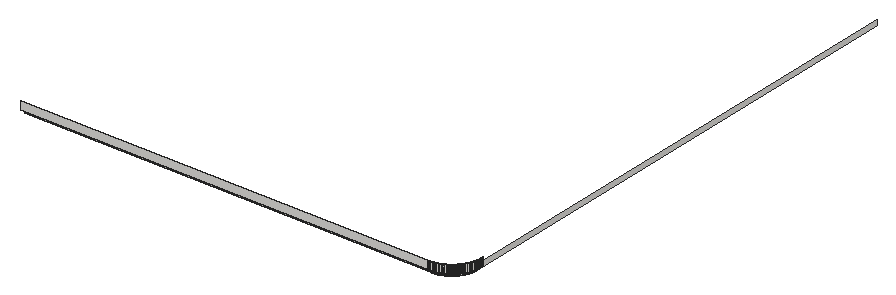
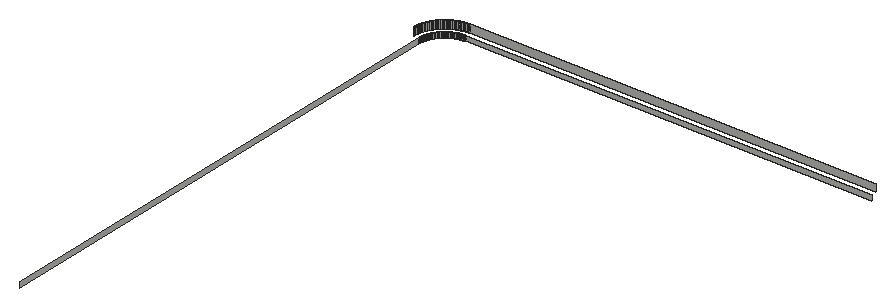
# SketchUp Ruby script. Lengths in inches.
U = 1.inch
M = Sketchup.active_model
def pt(a) = Geom::Point3d.new(a.map { |v| v * U })
def face(e, loops, mat)
  f = e.add_face(loops[0].map { |a| pt(a) })
  loops[1..].each { |l| e.add_face(l.map { |a| pt(a) }).erase! }
  f.material = f.back_material = mat if mat
  f
end
# faces: each face lists its corners as indices into pts; further lists are holes
def faces(e, pts, list, mat = nil) = list.each { |f| face(e, (f[0].is_a?(Array) ? f : [f]).map { |l| l.map { |i| pts[i] } }, mat) }
# xy, xz, yz: faces in a plane at the given z, y or x. An outline is a flat list of corners, or four numbers for a rectangle; further outlines are holes
def ring(l) = l.size == 4 ? [[l[0], l[1]], [l[2], l[1]], [l[2], l[3]], [l[0], l[3]]] : l.each_slice(2).to_a
def flat(e, list, mat, &to3) = list.each { |f| face(e, (f[0].is_a?(Array) ? f : [f]).map { |l| ring(l).map { |u, v| to3.(u, v) } }, mat) }
def xy(e, z, list, mat = nil) = flat(e, list, mat) { |x, y| [x, y, z] }
def xz(e, y, list, mat = nil) = flat(e, list, mat) { |x, z| [x, y, z] }
def yz(e, x, list, mat = nil) = flat(e, list, mat) { |y, z| [x, y, z] }
def lines(e, pts, list) = list.each { |a, b| e.add_line(pt(pts[a]), pt(pts[b])) }
# prism: a flat outline (further loops are holes) pulled along v
def prism(e, loops, v, mat = nil)
  f = face(e, loops, mat); d = Geom::Vector3d.new(v.map { |x| x * U })
  f.pushpull(f.normal.samedirection?(d) ? d.length : -d.length)
end
def box(e, o, s, mat = nil) = prism(e, [[o, [o[0] + s[0], o[1], o[2]], [o[0] + s[0], o[1] + s[1], o[2]], [o[0], o[1] + s[1], o[2]]]], [0, 0, s[2]], mat)
def at(x, y, z, deg = 0) = Geom::Transformation.translation(pt([x, y, z])) * Geom::Transformation.rotation(ORIGIN, Z_AXIS, deg.degrees)
def axes(o, x, y, z) = Geom::Transformation.new([*x, 0, *y, 0, *z, 0, *pt(o).to_a, 1])
def part(name) = M.definitions.add(name)
# library, detail: a bought-in or finely detailed component or shape, given as its bounding box
def library(name, o, s) = part(name).tap { |d| box(d.entities, o, s) }
def detail(e, o, s) = box(e.add_group.entities, o, s)
def put(e, d, t, mat = nil) = e.add_instance(d, t).tap { |i| i.material = mat if mat }
def group(e, t, mat = nil) = e.add_group.tap { |g| g.transformation = t; g.material = mat if mat }.entities
root = M.entities
M.materials.add("[Formica Graystone]").color = [224, 223, 219]
xz(root,229,[[18,424.82,174,427.82],[174,424.82,174.16,427.82],[174.16,424.82,174.3125,427.82]],"[Formica Graystone]")
xz(root,231,[[18,422.82,174,424.82],[174,422.82,174.13,424.82],[174.13,422.82,174.26,424.82]],"[Formica Graystone]")
xz(root,231.01,[[174.39,422.82,174.52,424.82]],"[Formica Graystone]")
yz(root,183.99,[[240.48,422.82,240.61,424.82]],"[Formica Graystone]")
yz(root,184,[[240.74,422.82,240.87,424.82],[240.87,422.82,241,424.82],[241,422.82,432,424.82]],"[Formica Graystone]")
yz(root,186,[[240.6875,424.82,240.84,427.82],[240.84,424.82,241,427.82]],"[Formica Graystone]")
p = [[174.39,231.01,422.82],[174.39,231.01,424.82],[174.26,231,424.82],[174.26,231,422.82],[174.65,231.02,422.82],[174.65,231.02,424.82],
  [174.52,231.01,424.82],[174.52,231.01,422.82],[174.78,231.03,422.82],[174.78,231.03,424.82],[174.92,231.04,422.82],[174.92,231.04,424.82],
  [175.05,231.05,422.82],[175.05,231.05,424.82],[175.18,231.07,422.82],[175.18,231.07,424.82],[175.31,231.09,422.82],[175.31,231.09,424.82],
  [175.43,231.1,422.82],[175.43,231.1,424.82],[175.5625,231.125,422.82],[175.5625,231.125,424.82],[175.69,231.14,422.82],[175.69,231.14,424.82],
  [175.82,231.17,422.82],[175.82,231.17,424.82],[175.95,231.19,422.82],[175.95,231.19,424.82],[176.08,231.22,422.82],[176.08,231.22,424.82],
  [176.21,231.25,422.82],[176.21,231.25,424.82],[176.33,231.28,422.82],[176.33,231.28,424.82],[176.46,231.31,422.82],[176.46,231.31,424.82],
  [176.59,231.34,422.82],[176.59,231.34,424.82],[176.71,231.375,422.82],[176.71,231.375,424.82],[176.84,231.41,422.82],[176.84,231.41,424.82],
  [176.97,231.45,422.82],[176.97,231.45,424.82],[177.09,231.49,422.82],[177.09,231.49,424.82],[177.21,231.53,422.82],[177.21,231.53,424.82],
  [177.34,231.57,422.82],[177.34,231.57,424.82],[177.46,231.62,422.82],[177.46,231.62,424.82],[177.58,231.66,422.82],[177.58,231.66,424.82],
  [177.71,231.71,422.82],[177.71,231.71,424.82],[177.83,231.76,422.82],[177.83,231.76,424.82],[177.95,231.8125,422.82],[177.95,231.8125,424.82],
  [178.07,231.86,422.82],[178.07,231.86,424.82],[178.1875,231.92,422.82],[178.1875,231.92,424.82],[178.31,231.97,422.82],[178.31,231.97,424.82],
  [178.42,232.03,422.82],[178.42,232.03,424.82],[178.54,232.09,422.82],[178.54,232.09,424.82],[178.66,232.15,422.82],[178.66,232.15,424.82],
  [178.77,232.21,422.82],[178.77,232.21,424.82],[178.89,232.28,422.82],[178.89,232.28,424.82],[179,232.34,422.82],[179,232.34,424.82],
  [179.11,232.41,422.82],[179.11,232.41,424.82],[179.22,232.47,422.82],[179.22,232.47,424.82],[179.34,232.54,422.82],[179.34,232.54,424.82],
  [179.45,232.61,422.82],[179.45,232.61,424.82],[179.56,232.69,422.82],[179.56,232.69,424.82],[179.66,232.76,422.82],[179.66,232.76,424.82],
  [179.77,232.83,422.82],[179.77,232.83,424.82],[179.88,232.91,422.82],[179.88,232.91,424.82],[179.98,232.99,422.82],[179.98,232.99,424.82],
  [180.09,233.07,422.82],[180.09,233.07,424.82],[180.19,233.15,422.82],[180.19,233.15,424.82],[180.29,233.23,422.82],[180.29,233.23,424.82],
  [180.39,233.3125,422.82],[180.39,233.3125,424.82],[180.49,233.4,422.82],[180.49,233.4,424.82],[180.59,233.48,422.82],[180.59,233.48,424.82],
  [180.69,233.57,422.82],[180.69,233.57,424.82],[180.79,233.66,422.82],[180.79,233.66,424.82],[180.88,233.75,422.82],[180.88,233.75,424.82],
  [180.98,233.84,422.82],[180.98,233.84,424.82],[181.07,233.93,422.82],[181.07,233.93,424.82],[181.16,234.02,422.82],[181.16,234.02,424.82],
  [181.25,234.12,422.82],[181.25,234.12,424.82],[181.34,234.21,422.82],[181.34,234.21,424.82],[181.43,234.31,422.82],[181.43,234.31,424.82],
  [181.52,234.41,422.82],[181.52,234.41,424.82],[181.6,234.51,422.82],[181.6,234.51,424.82],[181.6875,234.61,422.82],[181.6875,234.61,424.82],
  [181.77,234.71,422.82],[181.77,234.71,424.82],[181.85,234.81,422.82],[181.85,234.81,424.82],[181.93,234.91,422.82],[181.93,234.91,424.82],
  [182.01,235.02,422.82],[182.01,235.02,424.82],[182.09,235.12,422.82],[182.09,235.12,424.82],[182.17,235.23,422.82],[182.17,235.23,424.82],
  [182.24,235.34,422.82],[182.24,235.34,424.82],[182.31,235.44,422.82],[182.31,235.44,424.82],[182.39,235.55,422.82],[182.39,235.55,424.82],
  [182.46,235.66,422.82],[182.46,235.66,424.82],[182.53,235.78,422.82],[182.53,235.78,424.82],[182.59,235.89,422.82],[182.59,235.89,424.82],
  [182.66,236,422.82],[182.66,236,424.82],[182.72,236.11,422.82],[182.72,236.11,424.82],[182.79,236.23,422.82],[182.79,236.23,424.82],
  [182.85,236.34,422.82],[182.85,236.34,424.82],[182.91,236.46,422.82],[182.91,236.46,424.82],[182.97,236.58,422.82],[182.97,236.58,424.82],
  [183.03,236.69,422.82],[183.03,236.69,424.82],[183.08,236.8125,422.82],[183.08,236.8125,424.82],[183.14,236.93,422.82],[183.14,236.93,424.82],
  [183.1875,237.05,422.82],[183.1875,237.05,424.82],[183.24,237.17,422.82],[183.24,237.17,424.82],[183.29,237.29,422.82],[183.29,237.29,424.82],
  [183.34,237.42,422.82],[183.34,237.42,424.82],[183.38,237.54,422.82],[183.38,237.54,424.82],[183.43,237.66,422.82],[183.43,237.66,424.82],
  [183.47,237.79,422.82],[183.47,237.79,424.82],[183.51,237.91,422.82],[183.51,237.91,424.82],[183.55,238.03,422.82],[183.55,238.03,424.82],
  [183.59,238.16,422.82],[183.59,238.16,424.82],[183.625,238.29,422.82],[183.625,238.29,424.82],[183.66,238.41,422.82],[183.66,238.41,424.82],
  [183.69,238.54,422.82],[183.69,238.54,424.82],[183.72,238.67,422.82],[183.72,238.67,424.82],[183.75,238.79,422.82],[183.75,238.79,424.82],
  [183.78,238.92,422.82],[183.78,238.92,424.82],[183.81,239.05,422.82],[183.81,239.05,424.82],[183.83,239.18,422.82],[183.83,239.18,424.82],
  [183.86,239.31,422.82],[183.86,239.31,424.82],[183.875,239.4375,422.82],[183.875,239.4375,424.82],[183.9,239.57,422.82],[183.9,239.57,424.82],
  [183.91,239.69,422.82],[183.91,239.69,424.82],[183.93,239.82,422.82],[183.93,239.82,424.82],[183.95,239.95,422.82],[183.95,239.95,424.82],
  [183.96,240.08,422.82],[183.96,240.08,424.82],[183.97,240.22,422.82],[183.97,240.22,424.82],[183.98,240.35,422.82],[183.98,240.35,424.82],
  [183.99,240.48,422.82],[183.99,240.48,424.82],[184,240.74,422.82],[184,240.74,424.82],[183.99,240.61,424.82],[183.99,240.61,422.82],
  [174.3125,229,424.82],[174.47,229.01,424.82],[174.47,229.01,427.82],[174.3125,229,427.82],[174.63,229.02,424.82],[174.63,229.02,427.82],
  [174.78,229.03,424.82],[174.78,229.03,427.82],[174.94,229.04,424.82],[174.94,229.04,427.82],[175.1,229.05,424.82],[175.1,229.05,427.82],
  [175.25,229.07,424.82],[175.25,229.07,427.82],[175.41,229.08,424.82],[175.41,229.08,427.82],[175.57,229.1,424.82],[175.57,229.1,427.82],
  [175.72,229.125,424.82],[175.72,229.125,427.82],[175.88,229.15,424.82],[175.88,229.15,427.82],[176.03,229.17,424.82],[176.03,229.17,427.82],
  [176.1875,229.2,424.82],[176.1875,229.2,427.82],[176.34,229.23,424.82],[176.34,229.23,427.82],[176.49,229.26,424.82],[176.49,229.26,427.82],
  [176.65,229.3,424.82],[176.65,229.3,427.82],[176.8,229.33,424.82],[176.8,229.33,427.82],[176.95,229.37,424.82],[176.95,229.37,427.82],
  [177.11,229.41,424.82],[177.11,229.41,427.82],[177.26,229.45,424.82],[177.26,229.45,427.82],[177.41,229.49,424.82],[177.41,229.49,427.82],
  [177.56,229.54,424.82],[177.56,229.54,427.82],[177.71,229.59,424.82],[177.71,229.59,427.82],[177.86,229.64,424.82],[177.86,229.64,427.82],
  [178.01,229.6875,424.82],[178.01,229.6875,427.82],[178.15,229.74,424.82],[178.15,229.74,427.82],[178.3,229.8,424.82],[178.3,229.8,427.82],
  [178.45,229.85,424.82],[178.45,229.85,427.82],[178.59,229.91,424.82],[178.59,229.91,427.82],[178.74,229.97,424.82],[178.74,229.97,427.82],
  [178.88,230.04,424.82],[178.88,230.04,427.82],[179.02,230.1,424.82],[179.02,230.1,427.82],[179.17,230.17,424.82],[179.17,230.17,427.82],
  [179.31,230.24,424.82],[179.31,230.24,427.82],[179.45,230.31,424.82],[179.45,230.31,427.82],[179.59,230.38,424.82],[179.59,230.38,427.82],
  [179.73,230.45,424.82],[179.73,230.45,427.82],[179.86,230.53,424.82],[179.86,230.53,427.82],[180,230.61,424.82],[180,230.61,427.82],
  [180.14,230.6875,424.82],[180.14,230.6875,427.82],[180.27,230.77,424.82],[180.27,230.77,427.82],[180.4,230.85,424.82],[180.4,230.85,427.82],
  [180.54,230.9375,424.82],[180.54,230.9375,427.82],[180.67,231.02,424.82],[180.67,231.02,427.82],[180.8,231.11,424.82],[180.8,231.11,427.82],
  [180.93,231.2,424.82],[180.93,231.2,427.82],[181.05,231.29,424.82],[181.05,231.29,427.82],[181.18,231.38,424.82],[181.18,231.38,427.82],
  [181.31,231.48,424.82],[181.31,231.48,427.82],[181.43,231.58,424.82],[181.43,231.58,427.82],[181.55,231.67,424.82],[181.55,231.67,427.82],
  [181.67,231.77,424.82],[181.67,231.77,427.82],[181.79,231.875,424.82],[181.79,231.875,427.82],[181.91,231.98,424.82],[181.91,231.98,427.82],
  [182.03,232.08,424.82],[182.03,232.08,427.82],[182.15,232.1875,424.82],[182.15,232.1875,427.82],[182.26,232.3,424.82],[182.26,232.3,427.82],
  [182.375,232.4,424.82],[182.375,232.4,427.82],[182.49,232.51,424.82],[182.49,232.51,427.82],[182.6,232.625,424.82],[182.6,232.625,427.82],
  [182.7,232.74,424.82],[182.7,232.74,427.82],[182.8125,232.85,424.82],[182.8125,232.85,427.82],[182.92,232.97,424.82],[182.92,232.97,427.82],
  [183.02,233.09,424.82],[183.02,233.09,427.82],[183.125,233.21,424.82],[183.125,233.21,427.82],[183.23,233.33,424.82],[183.23,233.33,427.82],
  [183.33,233.45,424.82],[183.33,233.45,427.82],[183.42,233.57,424.82],[183.42,233.57,427.82],[183.52,233.69,424.82],[183.52,233.69,427.82],
  [183.62,233.82,424.82],[183.62,233.82,427.82],[183.71,233.95,424.82],[183.71,233.95,427.82],[183.8,234.07,424.82],[183.8,234.07,427.82],
  [183.89,234.2,424.82],[183.89,234.2,427.82],[183.98,234.33,424.82],[183.98,234.33,427.82],[184.0625,234.46,424.82],[184.0625,234.46,427.82],
  [184.15,234.6,424.82],[184.15,234.6,427.82],[184.23,234.73,424.82],[184.23,234.73,427.82],[184.3125,234.86,424.82],[184.3125,234.86,427.82],
  [184.39,235,424.82],[184.39,235,427.82],[184.47,235.14,424.82],[184.47,235.14,427.82],[184.55,235.27,424.82],[184.55,235.27,427.82],
  [184.62,235.41,424.82],[184.62,235.41,427.82],[184.69,235.55,424.82],[184.69,235.55,427.82],[184.76,235.69,424.82],[184.76,235.69,427.82],
  [184.83,235.83,424.82],[184.83,235.83,427.82],[184.9,235.98,424.82],[184.9,235.98,427.82],[184.96,236.12,424.82],[184.96,236.12,427.82],
  [185.03,236.26,424.82],[185.03,236.26,427.82],[185.09,236.41,424.82],[185.09,236.41,427.82],[185.15,236.55,424.82],[185.15,236.55,427.82],
  [185.2,236.7,424.82],[185.2,236.7,427.82],[185.26,236.85,424.82],[185.26,236.85,427.82],[185.3125,236.99,424.82],[185.3125,236.99,427.82],
  [185.36,237.14,424.82],[185.36,237.14,427.82],[185.41,237.29,424.82],[185.41,237.29,427.82],[185.46,237.44,424.82],[185.46,237.44,427.82],
  [185.51,237.59,424.82],[185.51,237.59,427.82],[185.55,237.74,424.82],[185.55,237.74,427.82],[185.59,237.89,424.82],[185.59,237.89,427.82],
  [185.63,238.05,424.82],[185.63,238.05,427.82],[185.67,238.2,424.82],[185.67,238.2,427.82],[185.7,238.35,424.82],[185.7,238.35,427.82],
  [185.74,238.51,424.82],[185.74,238.51,427.82],[185.77,238.66,424.82],[185.77,238.66,427.82],[185.8,238.8125,424.82],[185.8,238.8125,427.82],
  [185.83,238.97,424.82],[185.83,238.97,427.82],[185.85,239.12,424.82],[185.85,239.12,427.82],[185.875,239.28,424.82],[185.875,239.28,427.82],
  [185.9,239.43,424.82],[185.9,239.43,427.82],[185.92,239.59,424.82],[185.92,239.59,427.82],[185.93,239.75,424.82],[185.93,239.75,427.82],
  [185.95,239.9,424.82],[185.95,239.9,427.82],[185.96,240.06,424.82],[185.96,240.06,427.82],[185.97,240.22,424.82],[185.97,240.22,427.82],
  [185.98,240.37,424.82],[185.98,240.37,427.82],[185.99,240.53,424.82],[185.99,240.53,427.82],[186,240.6875,424.82],[186,240.6875,427.82],
  [174,231,424.82],[174,231,427.82],[184,241,424.82],[184,241,427.82]]
faces(root,p,[[0,1,2,3],[4,5,6,7],[8,9,5,4],[10,11,9,8],[12,13,11,10],[14,15,13,12],[16,17,15,14],[18,19,17,16],
  [20,21,19,18],[22,23,21,20],[24,25,23,22],[26,27,25,24],[28,29,27,26],[30,31,29,28],[32,33,31,30],[34,35,33,32],
  [36,37,35,34],[38,39,37,36],[40,41,39,38],[42,43,41,40],[44,45,43,42],[46,47,45,44],[48,49,47,46],[50,51,49,48],
  [52,53,51,50],[54,55,53,52],[56,57,55,54],[58,59,57,56],[60,61,59,58],[62,63,61,60],[64,65,63,62],[66,67,65,64],
  [68,69,67,66],[70,71,69,68],[72,73,71,70],[74,75,73,72],[76,77,75,74],[78,79,77,76],[80,81,79,78],[82,83,81,80],
  [84,85,83,82],[86,87,85,84],[88,89,87,86],[90,91,89,88],[92,93,91,90],[94,95,93,92],[96,97,95,94],[98,99,97,96],
  [100,101,99,98],[102,103,101,100],[104,105,103,102],[106,107,105,104],[108,109,107,106],[110,111,109,108],[112,113,111,110],[114,115,113,112],
  [116,117,115,114],[118,119,117,116],[120,121,119,118],[122,123,121,120],[124,125,123,122],[126,127,125,124],[128,129,127,126],[130,131,129,128],
  [132,133,131,130],[134,135,133,132],[136,137,135,134],[138,139,137,136],[140,141,139,138],[142,143,141,140],[144,145,143,142],[146,147,145,144],
  [148,149,147,146],[150,151,149,148],[152,153,151,150],[154,155,153,152],[156,157,155,154],[158,159,157,156],[160,161,159,158],[162,163,161,160],
  [164,165,163,162],[166,167,165,164],[168,169,167,166],[170,171,169,168],[172,173,171,170],[174,175,173,172],[176,177,175,174],[178,179,177,176],
  [180,181,179,178],[182,183,181,180],[184,185,183,182],[186,187,185,184],[188,189,187,186],[190,191,189,188],[192,193,191,190],[194,195,193,192],
  [196,197,195,194],[198,199,197,196],[200,201,199,198],[202,203,201,200],[204,205,203,202],[206,207,205,204],[208,209,207,206],[210,211,209,208],
  [212,213,211,210],[214,215,213,212],[216,217,215,214],[218,219,217,216],[220,221,219,218],[222,223,221,220],[224,225,223,222],[226,227,225,224],
  [228,229,227,226],[230,231,232,233],[234,235,236,237],[235,238,239,236],[238,240,241,239],[240,242,243,241],[242,244,245,243],[244,246,247,245],
  [246,248,249,247],[248,250,251,249],[250,252,253,251],[252,254,255,253],[254,256,257,255],[256,258,259,257],[258,260,261,259],[260,262,263,261],
  [262,264,265,263],[264,266,267,265],[266,268,269,267],[268,270,271,269],[270,272,273,271],[272,274,275,273],[274,276,277,275],[276,278,279,277],
  [278,280,281,279],[280,282,283,281],[282,284,285,283],[284,286,287,285],[286,288,289,287],[288,290,291,289],[290,292,293,291],[292,294,295,293],
  [294,296,297,295],[296,298,299,297],[298,300,301,299],[300,302,303,301],[302,304,305,303],[304,306,307,305],[306,308,309,307],[308,310,311,309],
  [310,312,313,311],[312,314,315,313],[314,316,317,315],[316,318,319,317],[318,320,321,319],[320,322,323,321],[322,324,325,323],[324,326,327,325],
  [326,328,329,327],[328,330,331,329],[330,332,333,331],[332,334,335,333],[334,336,337,335],[336,338,339,337],[338,340,341,339],[340,342,343,341],
  [342,344,345,343],[344,346,347,345],[346,348,349,347],[348,350,351,349],[350,352,353,351],[352,354,355,353],[354,356,357,355],[356,358,359,357],
  [358,360,361,359],[360,362,363,361],[362,364,365,363],[364,366,367,365],[366,368,369,367],[368,370,371,369],[370,372,373,371],[372,374,375,373],
  [374,376,377,375],[376,378,379,377],[378,380,381,379],[380,382,383,381],[382,384,385,383],[384,386,387,385],[386,388,389,387],[388,390,391,389],
  [390,392,393,391],[392,394,395,393],[394,396,397,395],[396,398,399,397],[398,400,401,399],[400,402,403,401],[402,404,405,403],[404,406,407,405],
  [406,408,409,407],[408,410,411,409],[410,412,413,411],[412,414,415,413],[414,416,417,415],[416,418,419,417],[418,420,421,419],[420,422,423,421],
  [422,424,425,423],[424,426,427,425],[426,428,429,427],[428,430,431,429],[430,432,433,431],[432,434,435,433],[434,436,437,435],[436,438,439,437],
  [438,440,441,439],[440,442,443,441],[442,444,445,443],[444,446,447,445],[446,448,449,447],[448,450,451,449],[450,452,453,451],[452,454,455,453],
  [454,456,457,455],[456,458,459,457],[458,460,461,459],[460,462,463,461],[462,464,465,463],[464,466,467,465]],"[Formica Graystone]")
lines(root,p,[[468,469],[470,471]])
